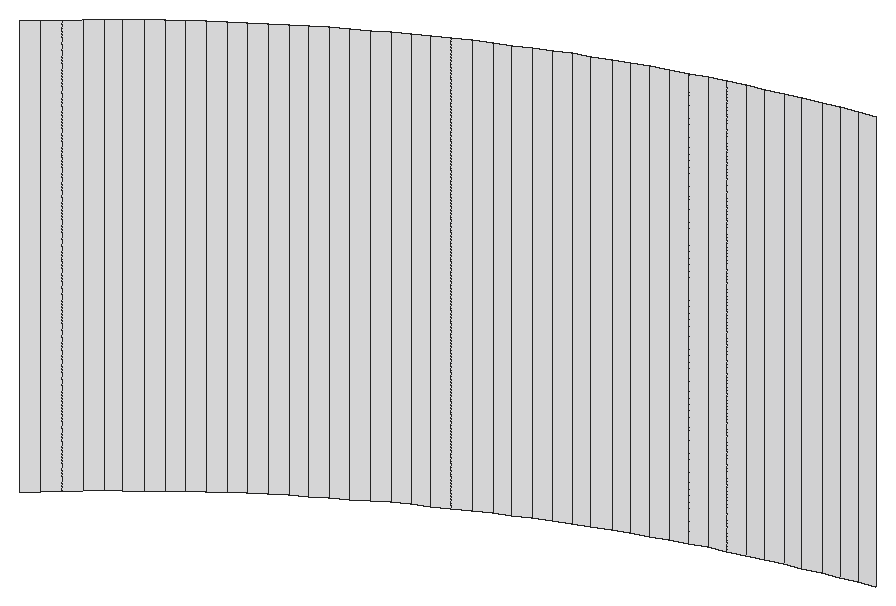
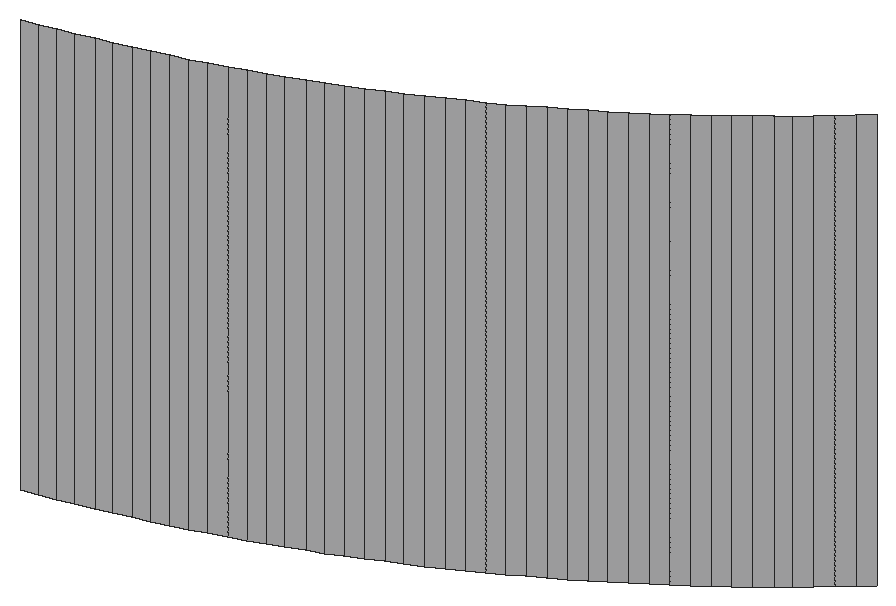
# SketchUp Ruby script. Lengths in inches.
U = 1.inch
M = Sketchup.active_model
def pt(a) = Geom::Point3d.new(a.map { |v| v * U })
def face(e, loops, mat)
  f = e.add_face(loops[0].map { |a| pt(a) })
  loops[1..].each { |l| e.add_face(l.map { |a| pt(a) }).erase! }
  f.material = f.back_material = mat if mat
  f
end
# faces: each face lists its corners as indices into pts; further lists are holes
def faces(e, pts, list, mat = nil) = list.each { |f| face(e, (f[0].is_a?(Array) ? f : [f]).map { |l| l.map { |i| pts[i] } }, mat) }
# xy, xz, yz: faces in a plane at the given z, y or x. An outline is a flat list of corners, or four numbers for a rectangle; further outlines are holes
def ring(l) = l.size == 4 ? [[l[0], l[1]], [l[2], l[1]], [l[2], l[3]], [l[0], l[3]]] : l.each_slice(2).to_a
def flat(e, list, mat, &to3) = list.each { |f| face(e, (f[0].is_a?(Array) ? f : [f]).map { |l| ring(l).map { |u, v| to3.(u, v) } }, mat) }
def xy(e, z, list, mat = nil) = flat(e, list, mat) { |x, y| [x, y, z] }
def xz(e, y, list, mat = nil) = flat(e, list, mat) { |x, z| [x, y, z] }
def yz(e, x, list, mat = nil) = flat(e, list, mat) { |y, z| [x, y, z] }
def lines(e, pts, list) = list.each { |a, b| e.add_line(pt(pts[a]), pt(pts[b])) }
# prism: a flat outline (further loops are holes) pulled along v
def prism(e, loops, v, mat = nil)
  f = face(e, loops, mat); d = Geom::Vector3d.new(v.map { |x| x * U })
  f.pushpull(f.normal.samedirection?(d) ? d.length : -d.length)
end
def box(e, o, s, mat = nil) = prism(e, [[o, [o[0] + s[0], o[1], o[2]], [o[0] + s[0], o[1] + s[1], o[2]], [o[0], o[1] + s[1], o[2]]]], [0, 0, s[2]], mat)
def at(x, y, z, deg = 0) = Geom::Transformation.translation(pt([x, y, z])) * Geom::Transformation.rotation(ORIGIN, Z_AXIS, deg.degrees)
def axes(o, x, y, z) = Geom::Transformation.new([*x, 0, *y, 0, *z, 0, *pt(o).to_a, 1])
def part(name) = M.definitions.add(name)
# library, detail: a bought-in or finely detailed component or shape, given as its bounding box
def library(name, o, s) = part(name).tap { |d| box(d.entities, o, s) }
def detail(e, o, s) = box(e.add_group.entities, o, s)
def put(e, d, t, mat = nil) = e.add_instance(d, t).tap { |i| i.material = mat if mat }
def group(e, t, mat = nil) = e.add_group.tap { |g| g.transformation = t; g.material = mat if mat }.entities
root = M.entities
M.materials.add("[Quartz Light Grey]").color = [251, 251, 252]
p = [[48.97,212.92,111.81],[49.09,213.02,111.81],[49.09,213.02,115.91],[48.97,212.92,115.91],[49.21,213.125,111.81],[49.21,213.125,115.91],
  [49.33,213.23,111.81],[49.33,213.23,115.91],[49.45,213.33,111.81],[49.45,213.33,115.91],[49.57,213.42,111.81],[49.57,213.42,115.91],
  [49.69,213.52,111.81],[49.69,213.52,115.91],[49.82,213.62,111.81],[49.82,213.62,115.91],[49.95,213.71,111.81],[49.95,213.71,115.91],
  [50.07,213.8,111.81],[50.07,213.8,115.91],[50.2,213.89,111.81],[50.2,213.89,115.91],[50.33,213.98,111.81],[50.33,213.98,115.91],
  [50.46,214.0625,111.81],[50.46,214.0625,115.91],[50.6,214.15,111.81],[50.6,214.15,115.91],[50.73,214.23,111.81],[50.73,214.23,115.91],
  [50.86,214.3125,111.81],[50.86,214.3125,115.91],[51,214.39,111.81],[51,214.39,115.91],[51.14,214.47,111.81],[51.14,214.47,115.91],
  [51.27,214.55,111.81],[51.27,214.55,115.91],[51.41,214.62,111.81],[51.41,214.62,115.91],[51.55,214.69,111.81],[51.55,214.69,115.91],
  [51.69,214.76,111.81],[51.69,214.76,115.91],[51.83,214.83,111.81],[51.83,214.83,115.91],[51.98,214.9,111.81],[51.98,214.9,115.91],
  [52.12,214.96,111.81],[52.12,214.96,115.91],[52.26,215.03,111.81],[52.26,215.03,115.91],[52.41,215.09,111.81],[52.41,215.09,115.91],
  [52.55,215.15,111.81],[52.55,215.15,115.91],[52.7,215.2,111.81],[52.7,215.2,115.91],[52.85,215.26,111.81],[52.85,215.26,115.91],
  [52.99,215.3125,111.81],[52.99,215.3125,115.91],[53.14,215.36,111.81],[53.14,215.36,115.91],[53.29,215.41,111.81],[53.29,215.41,115.91],
  [53.44,215.46,111.81],[53.44,215.46,115.91],[53.59,215.51,111.81],[53.59,215.51,115.91],[53.74,215.55,111.81],[53.74,215.55,115.91],
  [53.89,215.59,111.81],[53.89,215.59,115.91],[54.05,215.63,111.81],[54.05,215.63,115.91],[54.2,215.67,111.81],[54.2,215.67,115.91],
  [54.35,215.7,111.81],[54.35,215.7,115.91],[54.51,215.74,111.81],[54.51,215.74,115.91],[54.66,215.77,111.81],[54.66,215.77,115.91],
  [54.8125,215.8,111.81],[54.8125,215.8,115.91],[54.97,215.83,111.81],[54.97,215.83,115.91]]
faces(root,p,[[0,1,2,3],[1,4,5,2],[4,6,7,5],[6,8,9,7],[8,10,11,9],[10,12,13,11],[12,14,15,13],[14,16,17,15],
  [16,18,19,17],[18,20,21,19],[20,22,23,21],[22,24,25,23],[24,26,27,25],[26,28,29,27],[28,30,31,29],[30,32,33,31],
  [32,34,35,33],[34,36,37,35],[36,38,39,37],[38,40,41,39],[40,42,43,41],[42,44,45,43],[44,46,47,45],[46,48,49,47],
  [48,50,51,49],[50,52,53,51],[52,54,55,53],[54,56,57,55],[56,58,59,57],[58,60,61,59],[60,62,63,61],[62,64,65,63],
  [64,66,67,65],[66,68,69,67],[68,70,71,69],[70,72,73,71],[72,74,75,73],[74,76,77,75],[76,78,79,77],[78,80,81,79],
  [80,82,83,81],[82,84,85,83],[84,86,87,85]],"[Quartz Light Grey]")
